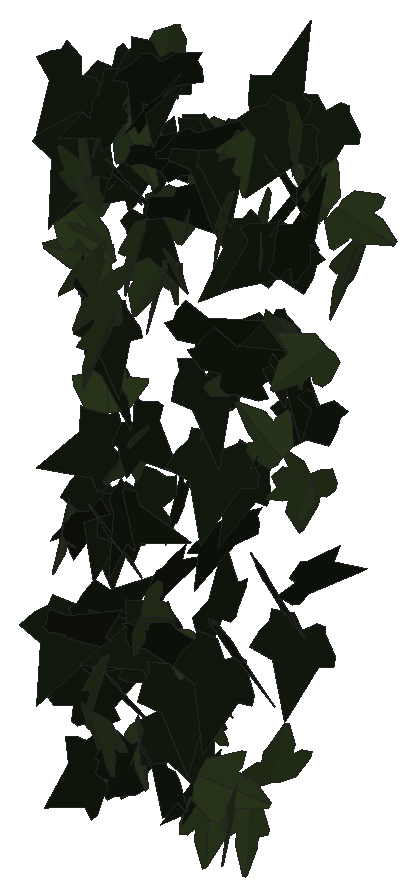
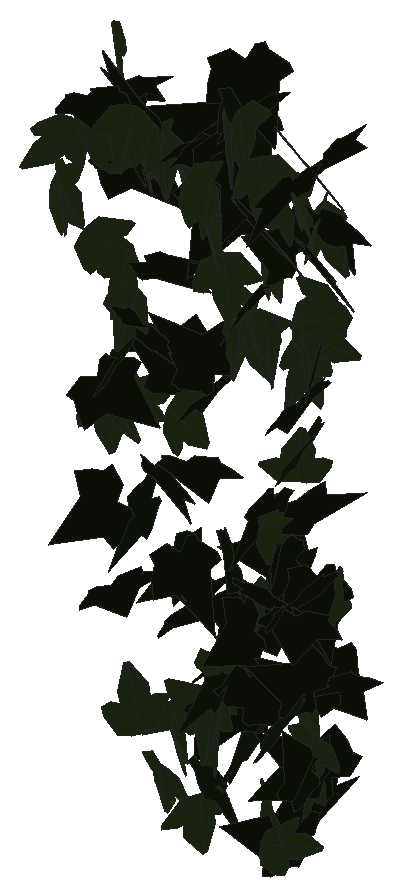
# SketchUp Ruby script. Lengths in inches.
U = 1.inch
M = Sketchup.active_model
def pt(a) = Geom::Point3d.new(a.map { |v| v * U })
def face(e, loops, mat)
  f = e.add_face(loops[0].map { |a| pt(a) })
  loops[1..].each { |l| e.add_face(l.map { |a| pt(a) }).erase! }
  f.material = f.back_material = mat if mat
  f
end
# faces: each face lists its corners as indices into pts; further lists are holes
def faces(e, pts, list, mat = nil) = list.each { |f| face(e, (f[0].is_a?(Array) ? f : [f]).map { |l| l.map { |i| pts[i] } }, mat) }
# xy, xz, yz: faces in a plane at the given z, y or x. An outline is a flat list of corners, or four numbers for a rectangle; further outlines are holes
def ring(l) = l.size == 4 ? [[l[0], l[1]], [l[2], l[1]], [l[2], l[3]], [l[0], l[3]]] : l.each_slice(2).to_a
def flat(e, list, mat, &to3) = list.each { |f| face(e, (f[0].is_a?(Array) ? f : [f]).map { |l| ring(l).map { |u, v| to3.(u, v) } }, mat) }
def xy(e, z, list, mat = nil) = flat(e, list, mat) { |x, y| [x, y, z] }
def xz(e, y, list, mat = nil) = flat(e, list, mat) { |x, z| [x, y, z] }
def yz(e, x, list, mat = nil) = flat(e, list, mat) { |y, z| [x, y, z] }
def lines(e, pts, list) = list.each { |a, b| e.add_line(pt(pts[a]), pt(pts[b])) }
# prism: a flat outline (further loops are holes) pulled along v
def prism(e, loops, v, mat = nil)
  f = face(e, loops, mat); d = Geom::Vector3d.new(v.map { |x| x * U })
  f.pushpull(f.normal.samedirection?(d) ? d.length : -d.length)
end
def box(e, o, s, mat = nil) = prism(e, [[o, [o[0] + s[0], o[1], o[2]], [o[0] + s[0], o[1] + s[1], o[2]], [o[0], o[1] + s[1], o[2]]]], [0, 0, s[2]], mat)
def at(x, y, z, deg = 0) = Geom::Transformation.translation(pt([x, y, z])) * Geom::Transformation.rotation(ORIGIN, Z_AXIS, deg.degrees)
def axes(o, x, y, z) = Geom::Transformation.new([*x, 0, *y, 0, *z, 0, *pt(o).to_a, 1])
def part(name) = M.definitions.add(name)
# library, detail: a bought-in or finely detailed component or shape, given as its bounding box
def library(name, o, s) = part(name).tap { |d| box(d.entities, o, s) }
def detail(e, o, s) = box(e.add_group.entities, o, s)
def put(e, d, t, mat = nil) = e.add_instance(d, t).tap { |i| i.material = mat if mat }
def group(e, t, mat = nil) = e.add_group.tap { |g| g.transformation = t; g.material = mat if mat }.entities
root = M.entities
M.materials.add("efeu1").color = [18, 25, 13]
M.materials.add("efeu2").color = [43, 57, 29]
c1 = part("ivyleaf_10")
p = [[0,0.5,-0.03],[-0.0625,2.02,-0.43],[-0.19,2.01,-0.46],[-0.54,1.05,-0.29],[-0.52,0.625,-0.18],[-0.83,0.76,-0.28],
  [-1.16,0.64,-0.33],[-1.15,0.33,-0.24],[-0.77,-0.39,0.02],[-0.3,-0.51,0.16],[0.04,-0.48,0.23],[-0.02,2.01,-0.4375],
  [-0.06,2.01,-0.43],[0.04,-0.49,0.23],[0.67,-0.49,0.14],[1.38,0.36,-0.2],[1.375,0.51,-0.24],[0.81,0.65,-0.19],
  [0.62,0.59,-0.15],[0.6,1.09,-0.28],[0.5,1.23,-0.31]]
faces(c1.entities,p,[[0,1,2,3,4,5,6,7,8,9,10],[11,12,0,13,14,15,16,17,18,19,20]],"efeu2")
c2 = part("ivyleaf_9")
p = [[1.54,2.16,1.25],[1.36,2.04,1.19],[-0.21,0.99,0.68],[-0.71,1.11,0.82],[-0.85,0.86,0.67],[-0.8,0.17,0.21],
  [-0.9,-0.01,0.1],[-0.67,-0.16,-0.02],[-0.08,-0.08,-0.05],[-0.03,-0.6,-0.4],[0.65,-0.88,-0.66],[0.83,-0.6,-0.49],
  [1.29,-0.42,-0.43],[1.8125,-0.07,-0.26],[1.21,0.44,0.15]]
faces(c2.entities,p,[[0,1,2,3,4,5,6,7,8,9,10,11,12,13,14]],"efeu1")
put(root,c1,axes([596.94,123.51,264.18],[0.27305,-1.12127,0.43947],[0.12601,-0.42155,-1.15384],[1.19771,0.29998,0.02121]))
put(root,c2,axes([595.99,124.04,243.86],[-0.20296,-0.59576,0.9813],[-0.33579,-0.92213,-0.62928],[1.09778,-0.3922,-0.01106]))
put(root,c2,axes([602.5,123.9,251.11],[-0.13816,-1.28206,0.33169],[-0.05092,-0.3281,-1.2894],[1.32329,-0.14648,-0.01499]))
put(root,c2,axes([600.5,123.79,249.51],[0.04781,-1.27209,0.07864],[0.16294,-0.07195,-1.26292],[1.26406,0.05739,0.15981]))
put(root,c2,axes([595.17,124.18,274.42],[-0.34558,-0.87945,0.61497],[-0.18363,-0.58808,-0.94419],[1.05731,-0.38958,0.03702]))
put(root,c1,axes([596.25,123.17,270.6],[-0.75885,-0.02382,0.91956],[-0.91981,0.0069,-0.75889],[0.00984,-1.19222,-0.02277]))
put(root,c1,axes([596.67,123.74,248.92],[0.42581,-1.02587,0.36752],[0.18485,-0.32086,-1.1098],[1.07392,0.46198,0.0453]))
put(root,c2,axes([599.48,124.2,245.23],[0.07296,-0.79141,0.86504],[0.23272,-0.8397,-0.78785],[1.14912,0.2203,0.10463]))
put(root,c1,axes([607.125,123.9,266.4],[-0.59909,-0.43431,0.86331],[-0.53981,-0.69212,-0.72278],[0.80159,-0.79068,0.15848]))
put(root,c2,axes([602.83,123.41,252.77],[1.03151,-0.60704,0.03],[0.02289,-0.02025,-1.19687],[0.60735,1.03175,-0.00584]))
put(root,c1,axes([602.93,124.03,245.04],[0.5828,-0.71904,0.76407],[0.52626,-0.5558,-0.92445],[0.90767,0.78393,0.04539]))
put(root,c2,axes([595.1,124.1,250.09],[-0.75889,-0.90505,0.01312],[-0.00396,-0.01379,-1.1811],[0.90513,-0.75888,0.00583]))
put(root,c2,axes([605.73,123.87,270.81],[0.12266,0.244,-1.19804],[-0.56533,-1.0563,-0.27301],[-1.08409,0.57844,0.00681]))
put(root,c1,axes([602.64,124,271.375],[0.58502,-0.92526,0.45871],[0.29219,-0.35736,-1.09347],[0.99053,0.65189,0.05163]))
put(root,c1,axes([598.23,124.02,268.55],[0.36446,-1.01048,0.47552],[0.30248,-0.39219,-1.06523],[1.07503,0.45293,0.13851]))
put(root,c2,axes([599.77,123.54,276.86],[0.17598,0.97332,-0.77439],[-0.13625,-0.76231,-0.9891],[-1.23632,0.22255,-0.00123]))
put(root,c2,axes([595.15,123.57,249.98],[0.98047,0.49921,-0.2946],[0.22713,0.20171,1.09774],[0.5333,-1.0037,0.07409]))
put(root,c2,axes([606.64,122.99,270.71],[-0.07297,-0.38498,1.2195],[0.60651,1.06495,0.37248],[-1.12585,0.59866,0.12162]))
put(root,c2,axes([597.28,124.41,256.15],[0.102,-0.03313,-1.17115],[0.96242,-0.66805,0.10272],[-0.66816,-0.96732,-0.03082]))
put(root,c2,axes([596.74,124.39,254.44],[0.96915,-0.49051,-0.43138],[0.39665,-0.17132,1.08594],[-0.519,-1.0469,0.02441]))
put(root,c2,axes([597.5,123.77,274.12],[-1.05654,0.57307,0.20236],[-0.17611,0.09972,-1.20195],[-0.58167,-1.07112,-0.00364]))
put(root,c1,axes([594.49,124.4,254.54],[-0.28447,0.68872,-0.88462],[0.07073,-0.89981,-0.72329],[-1.11888,-0.23199,0.17918]))
put(root,c2,axes([599.45,123.3,251.66],[1.15305,0.53657,-0.16756],[-0.14843,-0.07818,-1.27176],[-0.54218,1.16254,-0.00818]))
put(root,c1,axes([602.61,123.18,246.19],[0.23989,0.45907,1.08431],[0.57057,0.92267,-0.51687],[-1.03002,0.61803,-0.03377]))
put(root,c2,axes([595.34,124.34,271.71],[-1.15131,-0.41076,-0.45317],[0.42494,0.15754,-1.22238],[0.4399,-1.22722,-0.00524]))
put(root,c1,axes([604.11,124.57,271.55],[0.50137,-0.6935,0.82637],[0.62502,-0.556,-0.84582],[0.8793,0.79064,0.13003]))
put(root,c1,axes([599.19,123.28,252.36],[-0.01636,-0.60966,-1.0137],[0.09329,1.00997,-0.60892],[1.17922,-0.08836,0.03411]))
put(root,c1,axes([596.07,123.87,270.13],[-0.48169,1.05831,-0.15975],[-0.08918,0.13489,1.1625],[1.06657,0.48924,0.02506]))
put(root,c2,axes([596.0625,124.97,257.92],[-0.46478,-0.43933,0.94732],[-0.64252,-0.69708,-0.63851],[0.82316,-0.79216,0.03649]))
put(root,c1,axes([595.94,123.9375,266.57],[-0.20453,-1.11241,-0.40418],[0.03326,0.40461,-1.13041],[1.18309,-0.20369,-0.03809]))
put(root,c2,axes([600.65,123.375,273.11],[0.37377,1.11165,-0.63344],[0.10638,0.63063,1.16949],[1.27503,-0.37849,0.08812]))
put(root,c2,axes([600.125,124.16,247.53],[-0.25926,-0.77181,-0.90761],[0.28417,0.86198,-0.81419],[1.15702,-0.38465,-0.00341]))
put(root,c2,axes([601.09,124.77,273.45],[0.1179,-1.23943,-0.01792],[-0.0224,0.01587,-1.24485],[1.23936,0.1182,-0.02079]))
put(root,c2,axes([599.44,123.85,275.14],[-0.37036,1.26206,-0.0771],[0.0186,-0.07489,-1.31528],[-1.26428,-0.37081,0.00323]))
put(root,c1,axes([606.13,123.92,275.98],[0.61544,-0.66524,-0.76576],[-0.36937,0.68721,-0.89387],[0.94472,0.70206,0.14936]))
put(root,c2,axes([606.1,124.16,272.99],[-0.65914,1.03517,0.04247],[-0.02445,0.03478,-1.22721],[-1.03576,-0.65959,0.00194]))
put(root,c1,axes([598.72,124.77,266.39],[0.66771,-0.95438,0.07013],[0.04174,-0.05639,-1.16476],[0.95605,0.66901,0.00188]))
put(root,c1,axes([595.94,124.38,245.96],[-1.14853,0.37342,-0.02742],[0.03068,0.0057,-1.20762],[-0.37316,-1.14884,-0.0149]))
put(root,c1,axes([596.24,124.18,265.15],[-0.22597,-0.99732,-0.62733],[0.16663,0.60529,-1.02231],[1.16637,-0.27969,0.02451]))
put(root,c2,axes([604.17,124.27,255.51],[1.02806,-0.31088,-0.48295],[-0.45274,0.1707,-1.07363],[0.35343,1.12295,0.0295]))
put(root,c2,axes([596.78,124.36,255.45],[0.50932,0.08396,-1.03386],[0.78172,0.72598,0.44406],[0.68179,-0.89511,0.26318]))
put(root,c2,axes([598.32,125.23,275.73],[-0.06963,-1.17881,0.07972],[-0.00061,-0.07982,-1.18086],[1.18151,-0.06951,0.00409]))
put(root,c1,axes([595.96,124.96,272.74],[0.49482,-0.99019,0.21228],[0.08807,-0.19329,-1.10692],[1.00885,0.50254,-0.00749]))
put(root,c1,axes([606.05,124.83,259.96],[-0.5033,-1.08122,0.11806],[-0.04703,-0.10834,-1.19262],[1.08663,-0.50549,0.00307]))
put(root,c2,axes([600.15,123.99,270.85],[0.86592,0.95595,0.02826],[0.01675,0.02296,-1.28983],[-0.95622,0.86608,0.003]))
put(root,c2,axes([604.6875,125.45,272.4],[0.0354,-0.69826,0.98523],[0.52868,-0.87721,-0.64069],[1.0857,0.44992,0.27986]))
put(root,c2,axes([594.79,125.58,264.97],[-0.02057,-0.26072,1.14438],[-0.04572,-1.14351,-0.26134],[1.17281,-0.04915,0.00988]))
put(root,c1,axes([595.53,124.73,266.43],[0.22824,0.05034,-1.15018],[-1.14089,0.16707,-0.21909],[0.15433,1.16064,0.08142]))
put(root,c2,axes([598.95,124.16,272.64],[0.69718,0.89042,-0.05971],[-0.01861,-0.06124,-1.13065],[-0.89222,0.69704,-0.02307]))
put(root,c2,axes([595.4,124.47,255.02],[-0.05073,1.09817,-0.3424],[0.04848,-0.34039,-1.0989],[-1.14929,-0.06284,-0.03124]))
put(root,c1,axes([605.35,124.54,266.14],[-1.07709,0.43506,0.1365],[-0.12636,0.05162,-1.16164],[-0.43811,-1.08448,-0.00054]))
put(root,c1,axes([594.67,124.58,268],[0.72105,0.22948,0.8938],[0.82442,0.34942,-0.75478],[-0.41458,1.09394,0.05359]))
put(root,c2,axes([604.62,125.56,274.86],[-0.71847,-0.88693,0.24554],[-0.01079,-0.30337,-1.12739],[0.92023,-0.69603,0.17849]))
put(root,c2,axes([601.16,125.23,273.52],[0.06441,-1.26542,-0.13106],[0.12906,0.13705,-1.25983],[1.26563,0.05042,0.13513]))
put(root,c2,axes([595.43,125.05,270.37],[-1.10309,0.18462,-0.26502],[0.25997,-0.05214,-1.11841],[-0.19167,-1.13328,0.00828]))
put(root,c2,axes([596.14,125.13,270.07],[0.64131,-0.62728,0.72208],[0.59999,-0.41324,-0.89186],[0.74492,0.87288,0.09669]))
put(root,c2,axes([598.34,125.3,250.14],[-0.97354,-0.15093,0.56477],[-0.55681,-0.09474,-0.98515],[0.17805,-1.12151,0.00722]))
put(root,c1,axes([602.7,125.18,243.97],[1.09009,-0.27328,0.37392],[0.35409,-0.12459,-1.12334],[0.29853,1.14569,-0.03297]))
put(root,c2,axes([594.77,124.54,246.33],[0.01838,-0.04802,1.19794],[1.19096,0.13843,-0.01273],[-0.13779,1.19006,0.04982]))
put(root,c1,axes([596.86,125.26,272.07],[-0.81867,-0.01053,-0.84488],[0.74961,-0.55189,-0.71948],[-0.38989,-1.03897,0.39074]))
put(root,c2,axes([595.6,125.48,263.54],[0.17168,-1.15824,-0.04517],[-0.0066,0.04468,-1.17089],[1.1591,0.1718,0.00003]))
put(root,c1,axes([605.74,124.79,259.85],[0.41862,-0.24248,-1.02857],[-0.85817,0.56761,-0.48308],[0.61668,0.95448,0.02598]))
put(root,c2,axes([600.69,124.99,244.66],[-0.84168,0.82454,-0.07064],[0.0507,-0.04918,-1.17825],[-0.826,-0.8432,-0.00035]))
put(root,c1,axes([600.53,124.92,247.79],[-1.2123,0.31374,0.17194],[-0.1747,0.01097,-1.25181],[-0.31221,-1.22439,0.03284]))
put(root,c1,axes([604.11,125.0625,260.74],[0.63048,0.18419,0.91532],[-0.90751,-0.13873,0.65302],[0.21947,-1.10276,0.07073]))
put(root,c2,axes([600.33,125.61,262.19],[0.23133,-1.21427,0.00058],[-0.00046,-0.00068,-1.23611],[1.21427,0.23133,-0.00058]))
put(root,c2,axes([597.45,125.23,270.68],[-1.00504,0.46839,0.08214],[-0.07072,0.04271,-1.10879],[-0.47025,-1.00749,-0.00882]))
put(root,c2,axes([595.23,125.65,261.52],[0.52432,-0.9878,0.25663],[0.15182,-0.20981,-1.11779],[1.00924,0.54475,0.03483]))
put(root,c1,axes([595.9,125.06,260.11],[0.88754,0.7181,0.02468],[-0.02417,-0.00937,1.14164],[0.71812,-0.88783,0.00792]))
put(root,c2,axes([600.97,125.78,259.03],[-0.81672,-0.85302,-0.37641],[0.36754,0.16533,-1.17215],[0.85688,-0.88396,0.144]))
put(root,c1,axes([603.91,125.41,246.12],[-0.44598,-1.08893,0.01604],[0.02108,0.0087,1.17661],[-1.08884,0.44619,0.01621]))
put(root,c1,axes([597.92,125.65,266.17],[-0.54924,-0.90116,0.43278],[-0.24236,-0.35904,-1.05518],[0.96988,-0.60004,-0.01859]))
put(root,c1,axes([599.68,125.47,250.1],[1.13922,-0.12358,-0.14672],[-0.14453,0.02812,-1.14583],[0.12614,1.14828,0.01227]))
put(root,c1,axes([596.7,126.13,257.76],[-0.22117,0.40927,-1.00794],[-0.29935,-1.01174,-0.34513],[-1.04586,0.20304,0.31194]))
put(root,c2,axes([598.05,125.69,248.89],[-0.03419,0.10625,1.16073],[-1.1645,0.04688,-0.03859],[-0.05018,-1.16028,0.10473]))
put(root,c2,axes([604.65,126.03,252.22],[-0.35755,-1.12686,-0.05529],[0.02082,0.0514,-1.18222],[1.12802,-0.35813,0.00429]))
put(root,c2,axes([601.38,125.37,262.96],[0.11478,-0.1723,1.27264],[1.2405,-0.31577,-0.15463],[0.33234,1.23817,0.13766]))
put(root,c1,axes([602.84,125.78,273.42],[-0.61332,-0.93341,0.32222],[-0.03176,-0.36047,-1.10466],[0.98695,-0.59165,0.16469]))
put(root,c2,axes([595.4,124.89,250.17],[0.09379,-0.01048,1.07761],[0.95088,0.50983,-0.0778],[-0.50713,0.954,0.05342]))
put(root,c1,axes([594.61,125.63,248.36],[1.07671,-0.10545,0.3278],[0.33074,0.01727,-1.08083],[0.09582,1.12537,0.0473]))
put(root,c1,axes([596.14,126.27,243.34],[-0.24614,-0.15816,1.04049],[-0.23621,-1.03301,-0.2129],[1.02559,-0.27588,0.20069]))
put(root,c2,axes([598.34,125.59,271.53],[-1.03723,0.38549,0.13701],[-0.12176,0.06563,-1.10639],[-0.39058,-1.04418,-0.01896]))
put(root,c2,axes([594.98,126.3125,255.05],[-0.12709,-1.28295,0.25424],[-0.039,-0.25161,-1.28916],[1.30732,-0.13223,-0.01374]))
put(root,c1,axes([600.56,125.55,243.42],[0.46495,1.13959,-0.13152],[-0.15898,-0.07653,-1.22516],[-1.13609,0.47709,0.11762]))
put(root,c1,axes([600.1,125.82,271.59],[-0.64039,0.50121,-0.81827],[0.64127,-0.5083,-0.8132],[-0.71384,-0.90626,0.00355]))
put(root,c2,axes([597.34,125.57,268.24],[0.59954,-0.85816,-0.52457],[-0.2158,0.48672,-1.04288],[0.98236,0.63066,0.09106]))
put(root,c2,axes([599.87,125.68,263.62],[0.02951,-0.18475,1.15442],[1.11673,-0.33733,-0.08253],[0.34603,1.10443,0.16791]))
put(root,c1,axes([607.05,126.37,269.64],[0.29184,-0.99703,0.70379],[0.24741,-0.66028,-1.03797],[1.19507,0.38018,0.04302]))
put(root,c2,axes([601.52,125.08,252.34],[-0.97944,0.45716,-0.48242],[-0.43796,0.20228,1.08088],[0.49991,1.0729,0.00177]))
put(root,c1,axes([599.54,126.03,270.1],[0.6124,-0.96879,0.09099],[0.03985,-0.08245,-1.14607],[0.97224,0.61361,-0.01034]))
put(root,c1,axes([596.38,126.15,244.78],[0.64702,-0.31159,0.80284],[0.76593,-0.25085,-0.71463],[0.39369,1.00013,0.07088]))
put(root,c2,axes([599.3125,125.68,249.85],[1.01778,-0.46994,-0.30845],[-0.28139,0.12637,-1.12103],[0.48662,1.05596,-0.00311]))
put(root,c1,axes([600.04,125.09,246.54],[0.09307,-0.01007,-1.11887],[-0.26574,1.09041,-0.03192],[1.0869,0.26746,0.088]))
put(root,c2,axes([605.44,124.96,255.3],[0.51797,0.7125,0.80387],[0.48593,0.64049,-0.8808],[-0.95799,0.71012,-0.01213]))
put(root,c1,axes([605.92,125.79,272.0625],[0.61329,0.12514,1.01312],[-1.01702,-0.02699,0.61899],[0.088,-1.18398,0.09297]))
put(root,c1,axes([597.07,125.97,273.88],[-0.55742,-0.98208,-0.02114],[0.00645,0.02064,-1.12924],[0.98228,-0.55744,-0.00458]))
put(root,c2,axes([602.05,126.32,258.52],[-1.02859,-0.11762,-0.46549],[0.46546,0.02562,-1.03499],[0.11775,-1.12872,0.02502]))
put(root,c1,axes([597.83,126.26,275.98],[0.01045,-1.16504,0.22926],[0.36189,-0.21523,-1.11027],[1.13089,0.07964,0.35317]))
put(root,c1,axes([600.8125,126.64,261.625],[0.07929,-0.88728,0.75288],[0.07371,-0.74928,-0.8908],[1.16132,0.10814,0.00513]))
put(root,c2,axes([594.73,125.89,247.18],[1.04342,-0.39876,0.2221],[0.21395,-0.06223,-1.11688],[0.40318,1.06498,0.0179]))
put(root,c1,axes([607.34,125.65,271.95],[-0.47424,-0.59648,-0.83533],[0.74474,0.43327,-0.73219],[0.70634,-0.85729,0.21116]))
put(root,c1,axes([599.98,126.67,272.43],[-0.00018,-0.92288,0.72446],[0.16366,-0.71739,-0.91384],[1.16179,0.10092,0.12885]))
put(root,c2,axes([595.93,125.25,243.19],[0.11808,0.12643,1.20374],[1.00325,0.66637,-0.16841],[-0.6771,1.0094,-0.0396]))
put(root,c1,axes([603.8,125.92,265.53],[-1.07236,0.30855,-0.10582],[0.0996,-0.03652,-1.11584],[-0.31061,-1.07695,0.00752]))
put(root,c1,axes([602.07,126.13,273.65],[0.04154,-1.21034,-0.09889],[0.01192,0.09935,-1.21096],[1.21432,0.04043,0.01527]))
put(root,c2,axes([602.79,126.43,265.01],[-0.46816,-0.47412,-0.89524],[0.88176,0.29482,-0.61725],[0.49874,-0.96629,0.25093]))
put(root,c2,axes([604.77,126.68,261.96],[-0.12193,0.41848,-1.08834],[-0.00446,-1.09444,-0.42032],[-1.16602,-0.03957,0.11542]))
put(root,c2,axes([602.08,126.77,268.25],[-0.96757,-0.49524,0.21957],[-0.1684,-0.15222,-1.08542],[0.51489,-0.98043,0.05762]))
put(root,c2,axes([603.72,126.97,263.12],[0.27274,-1.00568,0.65559],[0.15382,-0.63748,-1.04189],[1.1906,0.31274,-0.01557]))
put(root,c2,axes([594.86,126.51,254.375],[-0.61999,-0.76027,-0.60995],[0.41491,0.44826,-0.98048],[0.88198,-0.74531,0.03248]))
put(root,c2,axes([595.46,126.05,273.96],[0.42255,-0.90025,-0.75192],[-0.19545,0.73401,-0.98864],[1.15656,0.45294,0.10764]))
put(root,c2,axes([596.68,125.78,258.8],[0.37098,-0.47658,-0.94765],[-0.47048,0.82586,-0.5995],[0.95069,0.59467,0.07311]))
put(root,c2,axes([594.81,125.9,246.61],[-0.18107,-0.57667,0.95215],[0.66693,0.71615,0.56058],[-0.89125,0.65307,0.22604]))
put(root,c1,axes([597.94,126.07,266.6],[-0.98302,0.58571,0.15816],[-0.13567,0.0813,-1.14429],[-0.59133,-0.99234,-0.0004]))
put(root,c1,axes([607.22,126.17,270.26],[0.45539,-0.97498,-0.46531],[-0.16786,0.43497,-1.07568],[1.0672,0.48445,0.02936]))
put(root,c1,axes([596.67,125.91,266.7],[0.67165,-0.54951,-0.7788],[-0.33224,0.75801,-0.82137],[0.89337,0.69503,0.28006]))
put(root,c2,axes([598.01,125.43,252.17],[0.22294,0.64113,0.94208],[0.37545,0.86501,-0.67753],[-1.07591,0.4347,-0.04123]))
put(root,c1,axes([598.61,126.47,269.125],[-0.98363,-0.48084,0.23605],[-0.20829,-0.11138,-1.09483],[0.4935,-1.0054,0.0084]))
put(root,c2,axes([597.125,126.69,254.89],[-0.90536,0.28035,0.55794],[-0.58923,-0.05838,-0.9268],[-0.20664,-1.06186,0.19826]))
put(root,c2,axes([598.68,125.72,255.29],[-0.09803,0.52806,0.95927],[-0.13426,0.95004,-0.5367],[-1.08675,-0.165,-0.02022]))
put(root,c2,axes([603.42,126.02,274.69],[-1.04204,0.79256,0.39181],[0.31205,-0.23695,1.3092],[0.82722,1.08776,-0.0003]))
put(root,c2,axes([595.12,127.08,249.47],[0.46233,-1.06208,0.29567],[0.1554,-0.25463,-1.15767],[1.09146,0.48614,0.03959]))
put(root,c2,axes([600.625,126.61,255.27],[-0.20242,0.99267,-0.67148],[0.13493,-0.65779,-1.0131],[-1.19083,-0.24327,-0.00065]))
put(root,c2,axes([605.05,127.02,274.95],[-0.56162,-0.93242,-0.28042],[0.15424,0.23445,-1.08844],[0.96138,-0.58232,0.0108]))
put(root,c1,axes([598.35,126.55,275.62],[0.8029,-0.84405,-0.21376],[-0.00259,0.28846,-1.14871],[0.87069,0.77919,0.1937]))
put(root,c1,axes([603.38,126.5,274.27],[-1.05328,-0.36926,-0.11006],[0.11178,0.01375,-1.11588],[0.36874,-1.05893,0.02389]))
